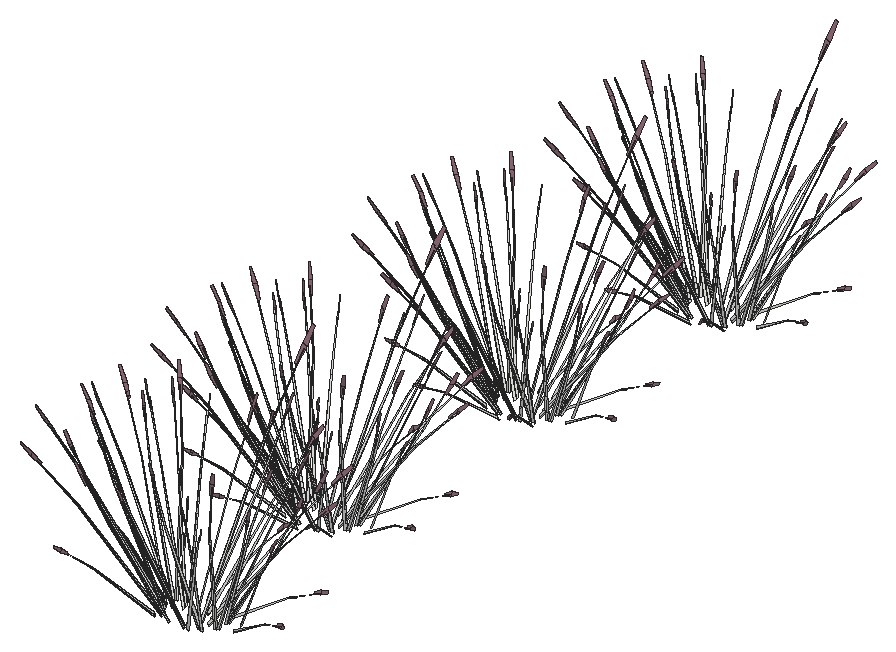
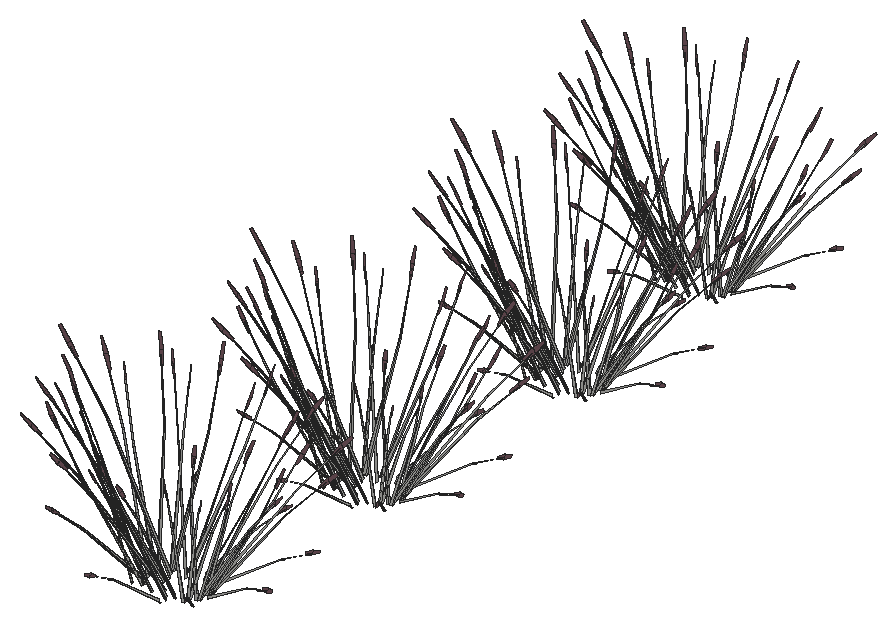
# SketchUp Ruby script. Lengths in inches.
U = 1.inch
M = Sketchup.active_model
def pt(a) = Geom::Point3d.new(a.map { |v| v * U })
def face(e, loops, mat)
  f = e.add_face(loops[0].map { |a| pt(a) })
  loops[1..].each { |l| e.add_face(l.map { |a| pt(a) }).erase! }
  f.material = f.back_material = mat if mat
  f
end
# faces: each face lists its corners as indices into pts; further lists are holes
def faces(e, pts, list, mat = nil) = list.each { |f| face(e, (f[0].is_a?(Array) ? f : [f]).map { |l| l.map { |i| pts[i] } }, mat) }
# xy, xz, yz: faces in a plane at the given z, y or x. An outline is a flat list of corners, or four numbers for a rectangle; further outlines are holes
def ring(l) = l.size == 4 ? [[l[0], l[1]], [l[2], l[1]], [l[2], l[3]], [l[0], l[3]]] : l.each_slice(2).to_a
def flat(e, list, mat, &to3) = list.each { |f| face(e, (f[0].is_a?(Array) ? f : [f]).map { |l| ring(l).map { |u, v| to3.(u, v) } }, mat) }
def xy(e, z, list, mat = nil) = flat(e, list, mat) { |x, y| [x, y, z] }
def xz(e, y, list, mat = nil) = flat(e, list, mat) { |x, z| [x, y, z] }
def yz(e, x, list, mat = nil) = flat(e, list, mat) { |y, z| [x, y, z] }
def lines(e, pts, list) = list.each { |a, b| e.add_line(pt(pts[a]), pt(pts[b])) }
# prism: a flat outline (further loops are holes) pulled along v
def prism(e, loops, v, mat = nil)
  f = face(e, loops, mat); d = Geom::Vector3d.new(v.map { |x| x * U })
  f.pushpull(f.normal.samedirection?(d) ? d.length : -d.length)
end
def box(e, o, s, mat = nil) = prism(e, [[o, [o[0] + s[0], o[1], o[2]], [o[0] + s[0], o[1] + s[1], o[2]], [o[0], o[1] + s[1], o[2]]]], [0, 0, s[2]], mat)
def at(x, y, z, deg = 0) = Geom::Transformation.translation(pt([x, y, z])) * Geom::Transformation.rotation(ORIGIN, Z_AXIS, deg.degrees)
def axes(o, x, y, z) = Geom::Transformation.new([*x, 0, *y, 0, *z, 0, *pt(o).to_a, 1])
def part(name) = M.definitions.add(name)
# library, detail: a bought-in or finely detailed component or shape, given as its bounding box
def library(name, o, s) = part(name).tap { |d| box(d.entities, o, s) }
def detail(e, o, s) = box(e.add_group.entities, o, s)
def put(e, d, t, mat = nil) = e.add_instance(d, t).tap { |i| i.material = mat if mat }
def group(e, t, mat = nil) = e.add_group.tap { |g| g.transformation = t; g.material = mat if mat }.entities
root = M.entities
M.materials.add("LightPink_Translucent").color = [144, 107, 117]
c1 = part("blade")
p = [[2.15,0.21,22],[0,0.17,0],[0.09,0.45,0],[2.18,0.31,22],[2.29,0.31,22],[0.38,0.45,0],
  [2.48,0.24,33],[2.49,0.24,33],[2.48,0.22,33]]
faces(c1.entities,p,[[0,1,2,3],[4,5,2,3],[6,3,4,7],[8,0,3,6]])
c2 = part("seeds")
p = [[0.3,-0.1,1.38],[-0.01,-0.03,1.59],[-0.01,-0.03,0.03],[0.14,-0.07,-0.07],[0.29,-0.03,3],[0.15,0.01,3.11]]
faces(c2.entities,p,[[0,1,2,3],[1,0,4,5]],"LightPink_Translucent")
c3 = part("blade with seeds")
put(c3.entities,c1,at(0,0,0))
put(c3.entities,c2,axes([2.4,0.25,30.99],[1.5799,-0.05474,1.17369],[-0.12525,1.92788,0.29478],[-0.07173,-0.02425,1.56792]))
put(root,c3,axes([54.17,551.18,46.53],[0.36946,-0.79643,-0.35414],[1.07787,0.23229,0.4572],[-0.09883,-0.32066,0.87481]))
put(root,c3,axes([54.98,552.24,45.875],[-0.22818,0.35597,1.71376],[-0.95725,-0.73667,0.13857],[0.43183,-0.45914,0.73262]))
put(root,c3,axes([54.65,551.6875,47.03],[-1.19922,0.48218,-0.1216],[-0.58932,-0.85579,-0.67495],[-0.15822,-0.36063,1.02557]))
put(root,c3,axes([57.14,552.77,47.03],[-1.34686,-0.05131,-0.1216],[0.03681,-0.97156,-0.67495],[0.09356,-0.37418,1.02557]))
put(root,c3,axes([57.05,552.15,46.53],[0.82919,-0.54528,-0.35414],[0.78493,0.62262,0.4572],[0.11943,-0.31634,0.87481]))
put(root,c3,axes([51.0625,551.47,46.53],[-0.18927,-0.83419,-0.35414],[1.08199,-0.22027,0.4572],[-0.29062,-0.23905,0.87481]))
put(root,c3,axes([48.73,552.6875,45.875],[0.45521,0.17844,1.71376],[-0.94204,0.74856,0.13857],[-0.58713,-0.33769,0.73262]))
put(root,c3,axes([48.65,551.04,46.72],[-0.26368,-0.00731,1.74944],[-0.83946,0.73103,-0.27667],[-0.44791,-0.14937,0.14031]))
put(root,c3,axes([58.61,554.68,47.03],[-1.1336,-0.57106,-0.1216],[0.65308,-0.827,-0.67495],[0.32027,-0.28747,1.02557]))
put(root,c3,axes([58.92,554.1,46.53],[1.06674,-0.14801,-0.35414],[0.28168,0.84611,0.4572],[0.30569,-0.22726,0.87481]))
put(root,c3,axes([48.56,552.94,46.53],[-0.69728,-0.64842,-0.35414],[0.79619,-0.61382,0.4572],[-0.40453,-0.09339,0.87481]))
put(root,c3,axes([62,555.44,46.72],[0.17006,-0.15775,1.74944],[-0.21766,-0.96766,-0.27667],[0.42669,-0.18347,0.14031]))
put(root,c3,axes([49.36,552.87,47.03],[-0.06562,1.05324,-0.1216],[-1.2424,-0.02879,-0.67495],[-0.4785,-0.07316,1.02557]))
put(root,c3,axes([58.65,556.91,47.03],[-0.6166,-0.93779,-0.1216],[1.09436,-0.46085,-0.67495],[0.46117,-0.12373,1.02557]))
put(root,c3,axes([47.77,554.32,45.875],[0.50831,-0.02346,1.71376],[-0.33721,1.01661,0.13857],[-0.72439,-0.06288,0.73262]))
put(root,c3,axes([59.3,556.53,46.53],[1.01846,0.28891,-0.35414],[-0.29705,0.84289,0.4572],[0.41005,-0.07729,0.87481]))
put(root,c3,axes([47.33,555.19,46.53],[-1.01846,-0.28891,-0.35414],[0.29705,-0.84289,0.4572],[-0.41005,0.07729,0.87481]))
put(root,c3,axes([56.52,555.49,45.875],[-0.50831,0.02346,1.71376],[0.33721,-1.01661,0.13857],[0.72439,0.06288,0.73262]))
put(root,c3,axes([46.68,555.75,46.72],[-0.20012,0.13446,1.74944],[0.01702,0.98243,-0.27667],[-0.45871,0.12776,0.14031]))
put(root,c3,axes([47.97,554.82,47.03],[0.6166,0.93779,-0.1216],[-1.09436,0.46085,-0.67495],[-0.46117,0.12373,1.02557]))
put(root,c3,axes([60.14,558.88,45.93],[-0.23455,-0.87059,-0.03492],[1.10861,-0.20015,-0.15832],[0.23151,0.05519,0.52218]))
put(root,c3,axes([57.27,558.86,47.03],[0.06562,-1.05324,-0.1216],[1.2424,0.02879,-0.67495],[0.4785,0.07316,1.02557]))
put(root,c3,axes([58.35,558.23,46.72],[0.26289,-0.01751,1.74944],[0.72108,-0.8046,-0.27667],[0.46761,0.10621,0.14031]))
put(root,c3,axes([47.98,556.11,45.875],[0.42521,-0.21906,1.71376],[0.35798,1.01226,0.13857],[-0.66754,0.22878,0.73262]))
put(root,c3,axes([58.07,558.79,46.53],[0.69728,0.64842,-0.35414],[-0.79619,0.61382,0.4572],[0.40453,0.09339,0.87481]))
put(root,c3,axes([47.7,557.62,46.53],[-1.06674,0.14801,-0.35414],[-0.28168,-0.84611,0.4572],[-0.30569,0.22726,0.87481]))
put(root,c3,axes([55.5625,557.125,45.875],[-0.45521,-0.17844,1.71376],[0.94204,-0.74856,0.13857],[0.58713,0.33769,0.73262]))
put(root,c3,axes([55.65,554.77,46.47],[-1.05895,-0.53811,1.38283],[1.11816,-0.83781,0.59665],[0.34166,0.5049,1.33663]))
put(root,c3,axes([48.02,557.05,47.03],[1.1336,0.57106,-0.1216],[-0.65308,0.827,-0.67495],[-0.32027,0.28747,1.02557]))
put(root,c3,axes([54.82,560,47.03],[0.73026,-0.88648,-0.1216],[1.05755,0.51071,-0.67495],[0.36761,0.25045,1.02557]))
put(root,c3,axes([49.54,556.79,45.875],[0.30609,-0.31822,1.71376],[0.77286,0.85893,0.13857],[-0.53009,0.39116,0.73262]))
put(root,c3,axes([49.3125,557.57,45.875],[0.22818,-0.35597,1.71376],[0.95725,0.73667,0.13857],[-0.43183,0.45914,0.73262]))
put(root,c3,axes([49.58,559.58,46.53],[-0.82919,0.54528,-0.35414],[-0.78493,-0.62262,0.4572],[-0.11943,0.31634,0.87481]))
put(root,c3,axes([46.72,559.42,46.72],[-0.03046,0.20495,1.74944],[0.86449,0.71297,-0.27667],[-0.22632,0.33716,0.14031]))
put(root,c3,axes([51.97,560.04,47.03],[1.19922,-0.48218,-0.1216],[0.58932,0.85579,-0.67495],[0.15822,0.36063,1.02557]))
put(root,c3,axes([53.6875,558.16,45.875],[-0.28013,-0.33252,1.71376],[1.29445,-0.27994,0.13857],[0.29256,0.52202,0.73262]))
put(root,c3,axes([52.45,560.54,46.53],[-0.36946,0.79643,-0.35414],[-1.07787,-0.23229,0.4572],[0.09883,0.32066,0.87481]))
put(root,c3,axes([51.4,558.33,45.875],[-0.02999,-0.3975,1.71376],[1.30002,0.26369,0.13857],[-0.08041,0.56647,0.73262]))
put(root,c3,axes([51.69,561.96,46.72],[0.15534,0.16677,1.74944],[1.25362,0.06552,-0.27667],[0.12606,0.3678,0.14031]))
put(root,c3,axes([46.78,590.48,45.875],[0.28013,0.33252,1.71376],[-1.29445,0.27994,0.13857],[-0.29256,-0.52202,0.73262]))
put(root,c3,axes([48.92,588.27,46.72],[-0.18744,-0.14521,1.74944],[-1.25089,0.09206,-0.27667],[-0.19964,-0.34731,0.14031]))
put(root,c3,axes([54.54,590.05,46.72],[-0.01183,-0.20612,1.74944],[-0.99913,-0.59572,-0.27667],[0.15447,-0.36112,0.14031]))
put(root,c3,axes([50.34,590.01,46.53],[0.36946,-0.79643,-0.35414],[1.07787,0.23229,0.4572],[-0.09883,-0.32066,0.87481]))
put(root,c3,axes([51.15,591.0625,45.875],[-0.22818,0.35597,1.71376],[-0.95725,-0.73667,0.13857],[0.43183,-0.45914,0.73262]))
put(root,c3,axes([50.82,590.51,47.03],[-1.19922,0.48218,-0.1216],[-0.58932,-0.85579,-0.67495],[-0.15822,-0.36063,1.02557]))
put(root,c3,axes([53.3125,591.59,47.03],[-1.34686,-0.05131,-0.1216],[0.03681,-0.97156,-0.67495],[0.09356,-0.37418,1.02557]))
put(root,c3,axes([53.22,590.97,46.53],[0.82919,-0.54528,-0.35414],[0.78493,0.62262,0.4572],[0.11943,-0.31634,0.87481]))
put(root,c3,axes([47.23,590.3,46.53],[-0.18927,-0.83419,-0.35414],[1.08199,-0.22027,0.4572],[-0.29062,-0.23905,0.87481]))
put(root,c3,axes([44.9,591.51,45.875],[0.45521,0.17844,1.71376],[-0.94204,0.74856,0.13857],[-0.58713,-0.33769,0.73262]))
put(root,c3,axes([44.82,589.87,46.72],[-0.26368,-0.00731,1.74944],[-0.83946,0.73103,-0.27667],[-0.44791,-0.14937,0.14031]))
put(root,c3,axes([54.78,593.51,47.03],[-1.1336,-0.57106,-0.1216],[0.65308,-0.827,-0.67495],[0.32027,-0.28747,1.02557]))
put(root,c3,axes([55.09,592.93,46.53],[1.06674,-0.14801,-0.35414],[0.28168,0.84611,0.4572],[0.30569,-0.22726,0.87481]))
put(root,c3,axes([44.73,591.77,46.53],[-0.69728,-0.64842,-0.35414],[0.79619,-0.61382,0.4572],[-0.40453,-0.09339,0.87481]))
put(root,c3,axes([58.17,594.27,46.72],[0.17006,-0.15775,1.74944],[-0.21766,-0.96766,-0.27667],[0.42669,-0.18347,0.14031]))
put(root,c3,axes([45.53,591.69,47.03],[-0.06562,1.05324,-0.1216],[-1.2424,-0.02879,-0.67495],[-0.4785,-0.07316,1.02557]))
put(root,c3,axes([54.82,595.74,47.03],[-0.6166,-0.93779,-0.1216],[1.09436,-0.46085,-0.67495],[0.46117,-0.12373,1.02557]))
put(root,c3,axes([43.94,593.14,45.875],[0.50831,-0.02346,1.71376],[-0.33721,1.01661,0.13857],[-0.72439,-0.06288,0.73262]))
put(root,c3,axes([55.47,595.36,46.53],[1.01846,0.28891,-0.35414],[-0.29705,0.84289,0.4572],[0.41005,-0.07729,0.87481]))
put(root,c3,axes([43.5,594.02,46.53],[-1.01846,-0.28891,-0.35414],[0.29705,-0.84289,0.4572],[-0.41005,0.07729,0.87481]))
put(root,c3,axes([52.69,594.32,45.875],[-0.50831,0.02346,1.71376],[0.33721,-1.01661,0.13857],[0.72439,0.06288,0.73262]))
put(root,c3,axes([42.85,594.58,46.72],[-0.20012,0.13446,1.74944],[0.01702,0.98243,-0.27667],[-0.45871,0.12776,0.14031]))
put(root,c3,axes([44.14,593.64,47.03],[0.6166,0.93779,-0.1216],[-1.09436,0.46085,-0.67495],[-0.46117,0.12373,1.02557]))
put(root,c3,axes([56.3125,597.71,45.93],[-0.23455,-0.87059,-0.03492],[1.10861,-0.20015,-0.15832],[0.23151,0.05519,0.52218]))
put(root,c3,axes([53.4375,597.68,47.03],[0.06562,-1.05324,-0.1216],[1.2424,0.02879,-0.67495],[0.4785,0.07316,1.02557]))
put(root,c3,axes([54.52,597.05,46.72],[0.26289,-0.01751,1.74944],[0.72108,-0.8046,-0.27667],[0.46761,0.10621,0.14031]))
put(root,c3,axes([44.15,594.93,45.875],[0.42521,-0.21906,1.71376],[0.35798,1.01226,0.13857],[-0.66754,0.22878,0.73262]))
put(root,c3,axes([54.24,597.61,46.53],[0.69728,0.64842,-0.35414],[-0.79619,0.61382,0.4572],[0.40453,0.09339,0.87481]))
put(root,c3,axes([43.87,596.45,46.53],[-1.06674,0.14801,-0.35414],[-0.28168,-0.84611,0.4572],[-0.30569,0.22726,0.87481]))
put(root,c3,axes([51.73,595.95,45.875],[-0.45521,-0.17844,1.71376],[0.94204,-0.74856,0.13857],[0.58713,0.33769,0.73262]))
put(root,c3,axes([51.82,593.6,46.47],[-1.05895,-0.53811,1.38283],[1.11816,-0.83781,0.59665],[0.34166,0.5049,1.33663]))
put(root,c3,axes([44.1875,595.87,47.03],[1.1336,0.57106,-0.1216],[-0.65308,0.827,-0.67495],[-0.32027,0.28747,1.02557]))
put(root,c3,axes([50.99,598.83,47.03],[0.73026,-0.88648,-0.1216],[1.05755,0.51071,-0.67495],[0.36761,0.25045,1.02557]))
put(root,c3,axes([45.71,595.62,45.875],[0.30609,-0.31822,1.71376],[0.77286,0.85893,0.13857],[-0.53009,0.39116,0.73262]))
put(root,c3,axes([45.48,596.4,45.875],[0.22818,-0.35597,1.71376],[0.95725,0.73667,0.13857],[-0.43183,0.45914,0.73262]))
put(root,c3,axes([45.75,598.41,46.53],[-0.82919,0.54528,-0.35414],[-0.78493,-0.62262,0.4572],[-0.11943,0.31634,0.87481]))
put(root,c3,axes([42.89,598.25,46.72],[-0.03046,0.20495,1.74944],[0.86449,0.71297,-0.27667],[-0.22632,0.33716,0.14031]))
put(root,c3,axes([48.14,598.87,47.03],[1.19922,-0.48218,-0.1216],[0.58932,0.85579,-0.67495],[0.15822,0.36063,1.02557]))
put(root,c3,axes([49.86,596.99,45.875],[-0.28013,-0.33252,1.71376],[1.29445,-0.27994,0.13857],[0.29256,0.52202,0.73262]))
put(root,c3,axes([48.625,599.37,46.53],[-0.36946,0.79643,-0.35414],[-1.07787,-0.23229,0.4572],[0.09883,0.32066,0.87481]))
put(root,c3,axes([47.57,597.15,45.875],[-0.02999,-0.3975,1.71376],[1.30002,0.26369,0.13857],[-0.08041,0.56647,0.73262]))
put(root,c3,axes([47.86,600.78,46.72],[0.15534,0.16677,1.74944],[1.25362,0.06552,-0.27667],[0.12606,0.3678,0.14031]))
put(root,c3,axes([49.57,639.49,45.875],[0.28013,0.33252,1.71376],[-1.29445,0.27994,0.13857],[-0.29256,-0.52202,0.73262]))
put(root,c3,axes([51.71,637.28,46.72],[-0.18744,-0.14521,1.74944],[-1.25089,0.09206,-0.27667],[-0.19964,-0.34731,0.14031]))
put(root,c3,axes([57.33,639.0625,46.72],[-0.01183,-0.20612,1.74944],[-0.99913,-0.59572,-0.27667],[0.15447,-0.36112,0.14031]))
put(root,c3,axes([53.13,639.02,46.53],[0.36946,-0.79643,-0.35414],[1.07787,0.23229,0.4572],[-0.09883,-0.32066,0.87481]))
put(root,c3,axes([53.95,640.07,45.875],[-0.22818,0.35597,1.71376],[-0.95725,-0.73667,0.13857],[0.43183,-0.45914,0.73262]))
put(root,c3,axes([53.61,639.52,47.03],[-1.19922,0.48218,-0.1216],[-0.58932,-0.85579,-0.67495],[-0.15822,-0.36063,1.02557]))
put(root,c3,axes([56.1,640.6,47.03],[-1.34686,-0.05131,-0.1216],[0.03681,-0.97156,-0.67495],[0.09356,-0.37418,1.02557]))
put(root,c3,axes([56.01,639.98,46.53],[0.82919,-0.54528,-0.35414],[0.78493,0.62262,0.4572],[0.11943,-0.31634,0.87481]))
put(root,c3,axes([50.02,639.31,46.53],[-0.18927,-0.83419,-0.35414],[1.08199,-0.22027,0.4572],[-0.29062,-0.23905,0.87481]))
put(root,c3,axes([47.7,640.52,45.875],[0.45521,0.17844,1.71376],[-0.94204,0.74856,0.13857],[-0.58713,-0.33769,0.73262]))
put(root,c3,axes([47.61,638.88,46.72],[-0.26368,-0.00731,1.74944],[-0.83946,0.73103,-0.27667],[-0.44791,-0.14937,0.14031]))
put(root,c3,axes([57.57,642.52,47.03],[-1.1336,-0.57106,-0.1216],[0.65308,-0.827,-0.67495],[0.32027,-0.28747,1.02557]))
put(root,c3,axes([57.89,641.94,46.53],[1.06674,-0.14801,-0.35414],[0.28168,0.84611,0.4572],[0.30569,-0.22726,0.87481]))
put(root,c3,axes([47.52,640.78,46.53],[-0.69728,-0.64842,-0.35414],[0.79619,-0.61382,0.4572],[-0.40453,-0.09339,0.87481]))
put(root,c3,axes([60.96,643.28,46.72],[0.17006,-0.15775,1.74944],[-0.21766,-0.96766,-0.27667],[0.42669,-0.18347,0.14031]))
put(root,c3,axes([48.32,640.7,47.03],[-0.06562,1.05324,-0.1216],[-1.2424,-0.02879,-0.67495],[-0.4785,-0.07316,1.02557]))
put(root,c3,axes([57.62,644.75,47.03],[-0.6166,-0.93779,-0.1216],[1.09436,-0.46085,-0.67495],[0.46117,-0.12373,1.02557]))
put(root,c3,axes([46.74,642.15,45.875],[0.50831,-0.02346,1.71376],[-0.33721,1.01661,0.13857],[-0.72439,-0.06288,0.73262]))
put(root,c3,axes([58.26,644.37,46.53],[1.01846,0.28891,-0.35414],[-0.29705,0.84289,0.4572],[0.41005,-0.07729,0.87481]))
put(root,c3,axes([46.29,643.03,46.53],[-1.01846,-0.28891,-0.35414],[0.29705,-0.84289,0.4572],[-0.41005,0.07729,0.87481]))
put(root,c3,axes([55.48,643.33,45.875],[-0.50831,0.02346,1.71376],[0.33721,-1.01661,0.13857],[0.72439,0.06288,0.73262]))
put(root,c3,axes([45.65,643.59,46.72],[-0.20012,0.13446,1.74944],[0.01702,0.98243,-0.27667],[-0.45871,0.12776,0.14031]))
put(root,c3,axes([46.93,642.65,47.03],[0.6166,0.93779,-0.1216],[-1.09436,0.46085,-0.67495],[-0.46117,0.12373,1.02557]))
put(root,c3,axes([59.1,646.72,45.93],[-0.23455,-0.87059,-0.03492],[1.10861,-0.20015,-0.15832],[0.23151,0.05519,0.52218]))
put(root,c3,axes([56.23,646.69,47.03],[0.06562,-1.05324,-0.1216],[1.2424,0.02879,-0.67495],[0.4785,0.07316,1.02557]))
put(root,c3,axes([57.3125,646.0625,46.72],[0.26289,-0.01751,1.74944],[0.72108,-0.8046,-0.27667],[0.46761,0.10621,0.14031]))
put(root,c3,axes([46.95,643.94,45.875],[0.42521,-0.21906,1.71376],[0.35798,1.01226,0.13857],[-0.66754,0.22878,0.73262]))
put(root,c3,axes([57.03,646.62,46.53],[0.69728,0.64842,-0.35414],[-0.79619,0.61382,0.4572],[0.40453,0.09339,0.87481]))
put(root,c3,axes([46.66,645.46,46.53],[-1.06674,0.14801,-0.35414],[-0.28168,-0.84611,0.4572],[-0.30569,0.22726,0.87481]))
put(root,c3,axes([54.52,644.96,45.875],[-0.45521,-0.17844,1.71376],[0.94204,-0.74856,0.13857],[0.58713,0.33769,0.73262]))
put(root,c3,axes([54.61,642.61,46.47],[-1.05895,-0.53811,1.38283],[1.11816,-0.83781,0.59665],[0.34166,0.5049,1.33663]))
put(root,c3,axes([46.98,644.88,47.03],[1.1336,0.57106,-0.1216],[-0.65308,0.827,-0.67495],[-0.32027,0.28747,1.02557]))
put(root,c3,axes([53.78,647.84,47.03],[0.73026,-0.88648,-0.1216],[1.05755,0.51071,-0.67495],[0.36761,0.25045,1.02557]))
put(root,c3,axes([48.5,644.625,45.875],[0.30609,-0.31822,1.71376],[0.77286,0.85893,0.13857],[-0.53009,0.39116,0.73262]))
put(root,c3,axes([48.27,645.41,45.875],[0.22818,-0.35597,1.71376],[0.95725,0.73667,0.13857],[-0.43183,0.45914,0.73262]))
put(root,c3,axes([48.54,647.42,46.53],[-0.82919,0.54528,-0.35414],[-0.78493,-0.62262,0.4572],[-0.11943,0.31634,0.87481]))
put(root,c3,axes([45.68,647.26,46.72],[-0.03046,0.20495,1.74944],[0.86449,0.71297,-0.27667],[-0.22632,0.33716,0.14031]))
put(root,c3,axes([50.93,647.875,47.03],[1.19922,-0.48218,-0.1216],[0.58932,0.85579,-0.67495],[0.15822,0.36063,1.02557]))
put(root,c3,axes([52.65,646,45.875],[-0.28013,-0.33252,1.71376],[1.29445,-0.27994,0.13857],[0.29256,0.52202,0.73262]))
put(root,c3,axes([51.42,648.38,46.53],[-0.36946,0.79643,-0.35414],[-1.07787,-0.23229,0.4572],[0.09883,0.32066,0.87481]))
put(root,c3,axes([50.36,646.16,45.875],[-0.02999,-0.3975,1.71376],[1.30002,0.26369,0.13857],[-0.08041,0.56647,0.73262]))
put(root,c3,axes([50.65,649.79,46.72],[0.15534,0.16677,1.74944],[1.25362,0.06552,-0.27667],[0.12606,0.3678,0.14031]))
put(root,c3,axes([54.11,683.8125,45.875],[0.28013,0.33252,1.71376],[-1.29445,0.27994,0.13857],[-0.29256,-0.52202,0.73262]))
put(root,c3,axes([56.25,681.61,46.72],[-0.18744,-0.14521,1.74944],[-1.25089,0.09206,-0.27667],[-0.19964,-0.34731,0.14031]))
put(root,c3,axes([61.87,683.39,46.72],[-0.01183,-0.20612,1.74944],[-0.99913,-0.59572,-0.27667],[0.15447,-0.36112,0.14031]))
put(root,c3,axes([57.67,683.35,46.53],[0.36946,-0.79643,-0.35414],[1.07787,0.23229,0.4572],[-0.09883,-0.32066,0.87481]))
put(root,c3,axes([58.49,684.4,45.875],[-0.22818,0.35597,1.71376],[-0.95725,-0.73667,0.13857],[0.43183,-0.45914,0.73262]))
put(root,c3,axes([58.15,683.85,47.03],[-1.19922,0.48218,-0.1216],[-0.58932,-0.85579,-0.67495],[-0.15822,-0.36063,1.02557]))
put(root,c3,axes([60.64,684.93,47.03],[-1.34686,-0.05131,-0.1216],[0.03681,-0.97156,-0.67495],[0.09356,-0.37418,1.02557]))
put(root,c3,axes([60.55,684.31,46.53],[0.82919,-0.54528,-0.35414],[0.78493,0.62262,0.4572],[0.11943,-0.31634,0.87481]))
put(root,c3,axes([54.5625,683.64,46.53],[-0.18927,-0.83419,-0.35414],[1.08199,-0.22027,0.4572],[-0.29062,-0.23905,0.87481]))
put(root,c3,axes([52.24,684.85,45.875],[0.45521,0.17844,1.71376],[-0.94204,0.74856,0.13857],[-0.58713,-0.33769,0.73262]))
put(root,c3,axes([52.15,683.21,46.72],[-0.26368,-0.00731,1.74944],[-0.83946,0.73103,-0.27667],[-0.44791,-0.14937,0.14031]))
put(root,c3,axes([62.11,686.85,47.03],[-1.1336,-0.57106,-0.1216],[0.65308,-0.827,-0.67495],[0.32027,-0.28747,1.02557]))
put(root,c3,axes([62.43,686.27,46.53],[1.06674,-0.14801,-0.35414],[0.28168,0.84611,0.4572],[0.30569,-0.22726,0.87481]))
put(root,c3,axes([52.06,685.11,46.53],[-0.69728,-0.64842,-0.35414],[0.79619,-0.61382,0.4572],[-0.40453,-0.09339,0.87481]))
put(root,c3,axes([65.5,687.6,46.72],[0.17006,-0.15775,1.74944],[-0.21766,-0.96766,-0.27667],[0.42669,-0.18347,0.14031]))
put(root,c3,axes([52.86,685.03,47.03],[-0.06562,1.05324,-0.1216],[-1.2424,-0.02879,-0.67495],[-0.4785,-0.07316,1.02557]))
put(root,c3,axes([62.16,689.07,47.03],[-0.6166,-0.93779,-0.1216],[1.09436,-0.46085,-0.67495],[0.46117,-0.12373,1.02557]))
put(root,c3,axes([51.28,686.48,45.875],[0.50831,-0.02346,1.71376],[-0.33721,1.01661,0.13857],[-0.72439,-0.06288,0.73262]))
put(root,c3,axes([62.8,688.7,46.53],[1.01846,0.28891,-0.35414],[-0.29705,0.84289,0.4572],[0.41005,-0.07729,0.87481]))
put(root,c3,axes([50.83,687.36,46.53],[-1.01846,-0.28891,-0.35414],[0.29705,-0.84289,0.4572],[-0.41005,0.07729,0.87481]))
put(root,c3,axes([60.02,687.66,45.875],[-0.50831,0.02346,1.71376],[0.33721,-1.01661,0.13857],[0.72439,0.06288,0.73262]))
put(root,c3,axes([50.1875,687.92,46.72],[-0.20012,0.13446,1.74944],[0.01702,0.98243,-0.27667],[-0.45871,0.12776,0.14031]))
put(root,c3,axes([51.47,686.98,47.03],[0.6166,0.93779,-0.1216],[-1.09436,0.46085,-0.67495],[-0.46117,0.12373,1.02557]))
put(root,c3,axes([63.64,691.05,45.93],[-0.23455,-0.87059,-0.03492],[1.10861,-0.20015,-0.15832],[0.23151,0.05519,0.52218]))
put(root,c3,axes([60.77,691.02,47.03],[0.06562,-1.05324,-0.1216],[1.2424,0.02879,-0.67495],[0.4785,0.07316,1.02557]))
put(root,c3,axes([61.85,690.39,46.72],[0.26289,-0.01751,1.74944],[0.72108,-0.8046,-0.27667],[0.46761,0.10621,0.14031]))
put(root,c3,axes([51.49,688.27,45.875],[0.42521,-0.21906,1.71376],[0.35798,1.01226,0.13857],[-0.66754,0.22878,0.73262]))
put(root,c3,axes([61.57,690.95,46.53],[0.69728,0.64842,-0.35414],[-0.79619,0.61382,0.4572],[0.40453,0.09339,0.87481]))
put(root,c3,axes([51.2,689.79,46.53],[-1.06674,0.14801,-0.35414],[-0.28168,-0.84611,0.4572],[-0.30569,0.22726,0.87481]))
put(root,c3,axes([59.0625,689.29,45.875],[-0.45521,-0.17844,1.71376],[0.94204,-0.74856,0.13857],[0.58713,0.33769,0.73262]))
put(root,c3,axes([59.15,686.9375,46.47],[-1.05895,-0.53811,1.38283],[1.11816,-0.83781,0.59665],[0.34166,0.5049,1.33663]))
put(root,c3,axes([51.52,689.21,47.03],[1.1336,0.57106,-0.1216],[-0.65308,0.827,-0.67495],[-0.32027,0.28747,1.02557]))
put(root,c3,axes([58.32,692.17,47.03],[0.73026,-0.88648,-0.1216],[1.05755,0.51071,-0.67495],[0.36761,0.25045,1.02557]))
put(root,c3,axes([53.04,688.95,45.875],[0.30609,-0.31822,1.71376],[0.77286,0.85893,0.13857],[-0.53009,0.39116,0.73262]))
put(root,c3,axes([52.8125,689.74,45.875],[0.22818,-0.35597,1.71376],[0.95725,0.73667,0.13857],[-0.43183,0.45914,0.73262]))
put(root,c3,axes([53.08,691.75,46.53],[-0.82919,0.54528,-0.35414],[-0.78493,-0.62262,0.4572],[-0.11943,0.31634,0.87481]))
put(root,c3,axes([50.22,691.58,46.72],[-0.03046,0.20495,1.74944],[0.86449,0.71297,-0.27667],[-0.22632,0.33716,0.14031]))
put(root,c3,axes([55.47,692.2,47.03],[1.19922,-0.48218,-0.1216],[0.58932,0.85579,-0.67495],[0.15822,0.36063,1.02557]))
put(root,c3,axes([57.1875,690.32,45.875],[-0.28013,-0.33252,1.71376],[1.29445,-0.27994,0.13857],[0.29256,0.52202,0.73262]))
put(root,c3,axes([55.96,692.71,46.53],[-0.36946,0.79643,-0.35414],[-1.07787,-0.23229,0.4572],[0.09883,0.32066,0.87481]))
put(root,c3,axes([54.9,690.49,45.875],[-0.02999,-0.3975,1.71376],[1.30002,0.26369,0.13857],[-0.08041,0.56647,0.73262]))
put(root,c3,axes([55.19,694.12,46.72],[0.15534,0.16677,1.74944],[1.25362,0.06552,-0.27667],[0.12606,0.3678,0.14031]))
